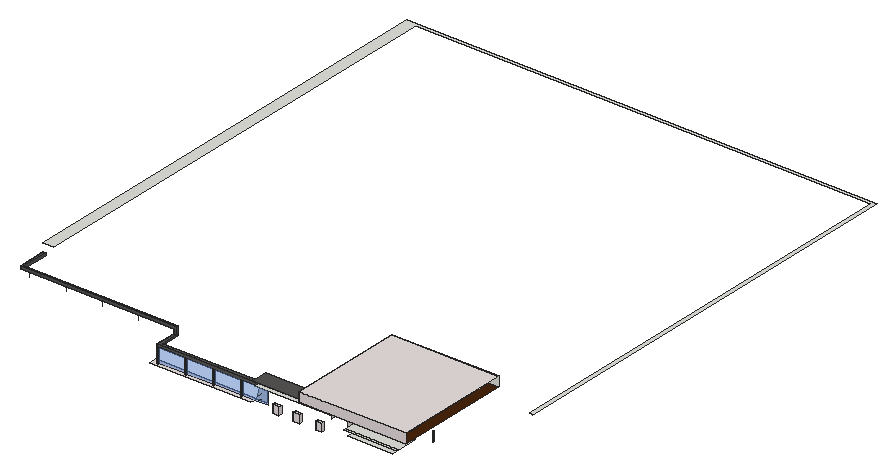
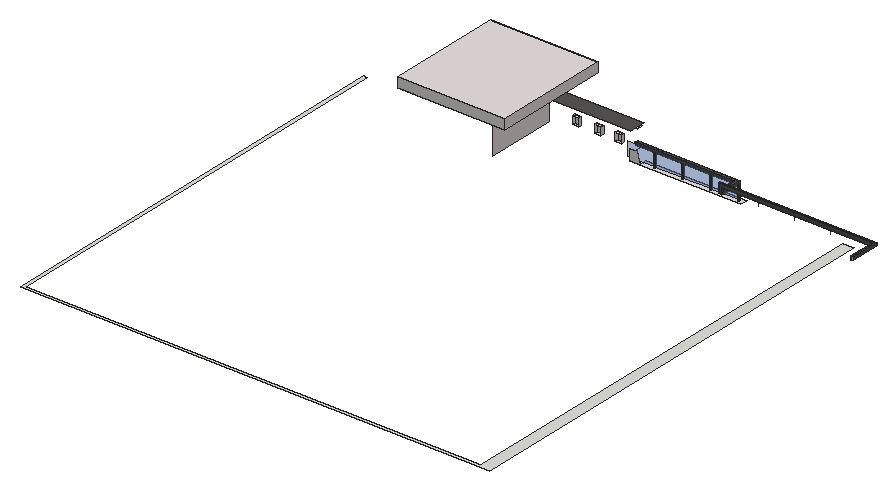
# SketchUp Ruby script. Lengths in inches.
U = 1.inch
M = Sketchup.active_model
def pt(a) = Geom::Point3d.new(a.map { |v| v * U })
def face(e, loops, mat)
  f = e.add_face(loops[0].map { |a| pt(a) })
  loops[1..].each { |l| e.add_face(l.map { |a| pt(a) }).erase! }
  f.material = f.back_material = mat if mat
  f
end
# faces: each face lists its corners as indices into pts; further lists are holes
def faces(e, pts, list, mat = nil) = list.each { |f| face(e, (f[0].is_a?(Array) ? f : [f]).map { |l| l.map { |i| pts[i] } }, mat) }
# xy, xz, yz: faces in a plane at the given z, y or x. An outline is a flat list of corners, or four numbers for a rectangle; further outlines are holes
def ring(l) = l.size == 4 ? [[l[0], l[1]], [l[2], l[1]], [l[2], l[3]], [l[0], l[3]]] : l.each_slice(2).to_a
def flat(e, list, mat, &to3) = list.each { |f| face(e, (f[0].is_a?(Array) ? f : [f]).map { |l| ring(l).map { |u, v| to3.(u, v) } }, mat) }
def xy(e, z, list, mat = nil) = flat(e, list, mat) { |x, y| [x, y, z] }
def xz(e, y, list, mat = nil) = flat(e, list, mat) { |x, z| [x, y, z] }
def yz(e, x, list, mat = nil) = flat(e, list, mat) { |y, z| [x, y, z] }
def lines(e, pts, list) = list.each { |a, b| e.add_line(pt(pts[a]), pt(pts[b])) }
# prism: a flat outline (further loops are holes) pulled along v
def prism(e, loops, v, mat = nil)
  f = face(e, loops, mat); d = Geom::Vector3d.new(v.map { |x| x * U })
  f.pushpull(f.normal.samedirection?(d) ? d.length : -d.length)
end
def box(e, o, s, mat = nil) = prism(e, [[o, [o[0] + s[0], o[1], o[2]], [o[0] + s[0], o[1] + s[1], o[2]], [o[0], o[1] + s[1], o[2]]]], [0, 0, s[2]], mat)
def at(x, y, z, deg = 0) = Geom::Transformation.translation(pt([x, y, z])) * Geom::Transformation.rotation(ORIGIN, Z_AXIS, deg.degrees)
def axes(o, x, y, z) = Geom::Transformation.new([*x, 0, *y, 0, *z, 0, *pt(o).to_a, 1])
def part(name) = M.definitions.add(name)
# library, detail: a bought-in or finely detailed component or shape, given as its bounding box
def library(name, o, s) = part(name).tap { |d| box(d.entities, o, s) }
def detail(e, o, s) = box(e.add_group.entities, o, s)
def put(e, d, t, mat = nil) = e.add_instance(d, t).tap { |i| i.material = mat if mat }
def group(e, t, mat = nil) = e.add_group.tap { |g| g.transformation = t; g.material = mat if mat }.entities
root = M.entities
M.materials.add("Generic\#1").color = [72, 38, 12]
M.materials.add("Generic\#2").color = [87, 84, 84]
M.materials.add("Generic\#9").color = [233, 223, 223]
M.materials.add("[Color M07]").color = [58, 58, 58]
M.materials.add("[Translucent Glass Blue]").color = [100, 149, 237]
M.materials["[Translucent Glass Blue]"].alpha = 0.5
xy(root,250.531,[[[209.664,120.9375,306.609,120.9375,306.609,124.118,296.245,123.803,296.244,123.791,296.175,123.625,296.066,123.482,295.924,123.373,295.758,123.305,295.58,123.281,295.402,123.305,295.236,123.373,295.094,123.482,294.984,123.625,294.916,123.791,294.892,123.969,294.916,124.147,294.984,124.3125,295.094,124.455,295.236,124.564,295.402,124.633,295.58,124.656,295.758,124.633,295.924,124.564,296.066,124.455,296.175,124.3125,296.244,124.147,296.267,123.969,296.245,123.803,306.609,124.118,306.609,127.4375,209.664,127.4375],[268.58,123.281,268.402,123.305,268.236,123.373,268.094,123.482,267.984,123.625,267.916,123.791,267.892,123.969,267.916,124.147,267.941,124.208,267.984,124.3125,268.094,124.455,268.236,124.564,268.402,124.633,268.58,124.656,268.758,124.633,268.924,124.564,269.066,124.455,269.175,124.3125,269.244,124.147,269.267,123.969,269.244,123.791,269.175,123.625,269.066,123.482,268.924,123.373,268.758,123.305],[241.767,123.281,241.589,123.305,241.424,123.373,241.281,123.482,241.172,123.625,241.103,123.791,241.08,123.969,241.103,124.147,241.172,124.3125,241.281,124.455,241.424,124.564,241.589,124.633,241.767,124.656,241.945,124.633,242.111,124.564,242.253,124.455,242.363,124.3125,242.431,124.147,242.455,123.969,242.431,123.791,242.363,123.625,242.253,123.482,242.111,123.373,241.945,123.305],[214.767,123.281,214.589,123.305,214.424,123.373,214.281,123.482,214.172,123.625,214.103,123.791,214.08,123.969,214.103,124.147,214.172,124.3125,214.281,124.455,214.424,124.564,214.589,124.633,214.767,124.656,214.945,124.633,215.111,124.564,215.253,124.455,215.363,124.3125,215.431,124.147,215.455,123.969,215.431,123.791,215.363,123.625,215.253,123.482,215.111,123.373,214.945,123.305]]],"Generic\#9")
xy(root,254.001,[[333.741,113.25,339.991,115.8125],[353.491,113.25,359.741,115.8125],[374.741,113.25,380.991,115.8125]],"Generic\#9")
xy(root,261.564,[[333.741,113.25,339.991,115.8125],[353.491,113.25,359.741,115.8125],[374.741,113.25,380.991,115.8125]],"Generic\#9")
xy(root,264.559,[[411.648,106.0625,454.828,113.125]])
xy(root,265.119,[[[214.101,123.115,214.101,123.807,214.103,123.791,214.172,123.625,214.281,123.482,214.424,123.373,214.589,123.305,214.767,123.281,214.945,123.305,241.589,123.305,241.767,123.281,241.945,123.305,242.363,123.305,242.363,123.625,242.431,123.791,242.455,123.969,242.431,124.147,242.363,124.3125,242.253,124.455,242.111,124.564,241.945,124.633,241.767,124.656,241.589,124.633,241.424,124.564,241.281,124.455,241.172,124.3125,215.363,124.3125,215.253,124.455,215.111,124.564,214.945,124.633,214.767,124.656,214.589,124.633,214.424,124.564,214.281,124.455,214.172,124.3125,214.103,124.147,214.101,124.13,214.101,145.287,217.038,145.287,217.038,126.052,311.912,126.052,311.912,123.115],[295.58,123.281,295.758,123.305,295.924,123.373,296.066,123.482,296.175,123.625,296.244,123.791,296.267,123.969,296.244,124.147,296.175,124.3125,296.066,124.455,295.924,124.564,295.758,124.633,295.58,124.656,295.402,124.633,295.236,124.564,295.094,124.455,294.984,124.3125,294.916,124.147,294.892,123.969,294.916,123.791,294.984,123.625,295.094,123.482,295.236,123.373,295.402,123.305],[268.58,123.281,268.758,123.305,268.924,123.373,269.066,123.482,269.175,123.625,269.244,123.791,269.267,123.969,269.244,124.147,269.175,124.3125,269.066,124.455,268.924,124.564,268.758,124.633,268.58,124.656,268.402,124.633,268.236,124.564,268.094,124.455,267.984,124.3125,267.916,124.147,267.892,123.969,267.916,123.791,267.984,123.625,268.094,123.482,268.236,123.373,268.402,123.305]],[311.912,123.115,312.403,126.052],[214.767,123.281,214.589,123.305,214.945,123.305],[241.767,123.281,241.589,123.305,241.945,123.305],[214.589,123.305,214.424,123.373,214.281,123.482,214.172,123.625,214.103,123.791,214.101,123.807,214.101,124.13,214.103,124.147,214.172,124.3125,214.281,124.455,214.424,124.564,214.589,124.633,214.767,124.656,214.945,124.633,215.111,124.564,215.253,124.455,215.363,124.3125,214.589,124.3125],
  [214.589,123.305,214.589,124.3125,215.363,124.3125,215.431,124.147,215.455,123.969,215.431,123.791,215.363,123.625,215.253,123.482,215.111,123.373,214.945,123.305],[214.945,123.305,215.111,123.373,215.253,123.482,215.363,123.625,215.431,123.791,215.455,123.969,215.431,124.147,215.363,124.3125,241.172,124.3125,241.103,124.147,241.08,123.969,241.103,123.791,241.172,123.625,241.281,123.482,241.424,123.373,241.589,123.305],[241.589,123.305,241.424,123.373,241.281,123.482,241.172,123.625,241.103,123.791,241.08,123.969,241.103,124.147,241.172,124.3125,242.363,124.3125,242.363,123.625,242.253,123.482,242.111,123.373,241.945,123.305],[241.945,123.305,242.111,123.373,242.253,123.482,242.363,123.625,242.363,123.305],[242.363,123.625,242.363,124.3125,242.431,124.147,242.455,123.969,242.431,123.791],
  [214.101,123.807,214.101,124.13,214.08,123.969],[241.172,124.3125,241.281,124.455,241.424,124.564,241.589,124.633,241.767,124.656,241.945,124.633,242.111,124.564,242.253,124.455,242.363,124.3125],[214.101,124.744,213.752,124.79,213.752,127.4375,214.101,127.4375]])
xy(root,267.247,[[214.294,123.307,214.294,143.159,217.231,143.159,217.231,126.245,312.403,126.245,312.403,123.307]],"Generic\#2")
xy(root,268.366,[[407.84,106.0625,458.635,108.375],[407.84,108.375,458.635,127.4375]])
xy(root,271.3125,[[75.429,143.428,75.607,143.451,75.773,143.52,75.915,143.629,76.025,143.771,76.093,143.937,76.117,144.115,76.093,144.293,76.025,144.459,75.915,144.601,75.773,144.711,75.607,144.779,75.429,144.803,75.251,144.779,75.086,144.711,74.943,144.601,74.834,144.459,74.765,144.293,74.742,144.115,74.765,143.937,74.834,143.771,74.943,143.629,75.086,143.52,75.251,143.451],[110.367,143.428,110.545,143.451,110.711,143.52,110.853,143.629,110.962,143.771,111.031,143.937,111.032,143.945,109.703,143.939,109.703,143.937,109.771,143.771,109.881,143.629,110.023,143.52,110.189,143.451],[145.179,143.428,145.357,143.451,145.523,143.52,145.665,143.629,145.775,143.771,145.843,143.937,145.867,144.115,145.866,144.118,144.492,144.112,144.515,143.937,144.584,143.771,144.693,143.629,144.836,143.52,145.001,143.451],[179.992,143.428,180.17,143.451,180.336,143.52,180.478,143.629,180.587,143.771,180.656,143.937,180.679,144.115,180.656,144.291,179.327,144.285,179.304,144.115,179.328,143.937,179.396,143.771,179.506,143.629,179.648,143.52,179.814,143.451],[214.992,143.428,215.17,143.451,215.336,143.52,215.478,143.629,215.587,143.771,215.656,143.937,215.679,144.115,215.656,144.293,215.587,144.459,215.478,144.601,215.336,144.711,215.17,144.779,214.992,144.803,214.955,144.798,214.814,144.779,214.648,144.711,214.506,144.601,214.396,144.459,214.328,144.293,214.304,144.115,214.328,143.937,214.396,143.771,214.506,143.629,214.648,143.52,214.814,143.451,214.955,143.433],
  [109.703,143.939,111.032,143.945,111.054,144.115,111.031,144.293,110.962,144.459,110.853,144.601,110.711,144.711,110.545,144.779,110.367,144.803,110.189,144.779,110.023,144.711,109.881,144.601,109.771,144.459,109.703,144.293,109.679,144.115],[144.492,144.112,145.866,144.118,145.843,144.293,145.775,144.459,145.665,144.601,145.523,144.711,145.357,144.779,145.179,144.803,145.001,144.779,144.836,144.711,144.693,144.601,144.584,144.459,144.515,144.293,144.492,144.115],[179.327,144.285,180.656,144.291,180.656,144.293,180.587,144.459,180.478,144.601,180.336,144.711,180.17,144.779,179.992,144.803,179.814,144.779,179.648,144.711,179.506,144.601,179.396,144.459,179.328,144.293]])
xy(root,272.627,[[317.954,111.75,393.08,115.8125],[393.08,111.75,394.852,115.8125]])
xy(root,276.252,[[315.959,111.75,394.852,127.4375]],"Generic\#2")
xy(root,281.899,[[67.114,170.6875,77.5625,170.6875,77.5625,605.125,515.25,605.125,515.25,194.75,518.6875,194.75,518.6875,607.4375,67.114,607.4375]])
xy(root,288.793,[[470.289,107.5625,470.852,108.375],[394.852,108.375,470.289,127.4375],[470.289,108.375,470.852,120.9375],[394.852,127.4375,470.289,194.75],[394.852,194.75,470.289,202.1875]])
xy(root,288.793,[[376.914,90.3125,376.914,202.1875,394.852,202.1875,394.852,108.375,470.289,108.375,470.289,107.5625,470.852,107.5625,470.852,120.9375,470.289,120.9375,470.289,202.1875,479.727,202.1875,479.727,90.3125]],"Generic\#1")
xy(root,297.793,[[376.914,90.3125,479.727,202.1875]],"Generic\#9")
xz(root,90.3125,[[376.914,288.793,479.727,297.793]],"Generic\#9")
xz(root,113.25,[[333.741,254.001,339.991,261.564],[353.491,254.001,359.741,261.564],[374.741,254.001,380.991,261.564]],"Generic\#9")
xz(root,127.4375,[[306.609,250.531,310.437,261.0625,316.414,261.0625,316.414,250.531]])
xz(root,143.159,[[214.294,267.247,214.294,271.308,67.114,271.308,67.114,274.245,217.231,274.245,217.231,267.247]],"Generic\#2")
xz(root,145.287,[[214.101,265.119,217.038,265.119,217.038,274.052,69.242,274.052,69.242,271.115,214.101,271.115]],"Generic\#2")
xz(root,170.75,[[69.242,271.115,69.242,274.052,67.114,274.245,67.114,271.308]])
xz(root,202.1875,[[376.914,288.793,479.727,297.793]])
yz(root,67.114,[[170.6875,271.308,170.75,274.245]])
yz(root,67.114,[[143.159,271.308,170.6875,274.245]],"Generic\#2")
yz(root,69.242,[[145.287,271.115,170.75,274.052]],"Generic\#2")
yz(root,312.403,[[123.115,265.119,123.237,266.469,123.307,267.247,126.245,267.247,126.175,266.469,126.052,265.119]])
yz(root,333.741,[[113.25,254.001,115.8125,261.564]],"Generic\#9")
yz(root,339.991,[[113.25,254.001,115.8125,261.564]],"Generic\#9")
yz(root,353.491,[[113.25,254.001,115.8125,261.564]],"Generic\#9")
yz(root,359.741,[[113.25,254.001,115.8125,261.564]],"Generic\#9")
yz(root,374.741,[[113.25,254.001,115.8125,261.564]],"Generic\#9")
yz(root,376.914,[[90.3125,288.793,202.1875,297.793]],"Generic\#9")
yz(root,380.991,[[113.25,254.001,115.8125,261.564]],"Generic\#9")
yz(root,394.852,[[108.375,272.627,111.75,276.252],[111.75,272.627,127.4375,276.252]])
yz(root,394.852,[[127.4375,256.5625,127.4375,276.252,108.375,276.252,108.375,288.793,194.75,288.793,194.75,256.5625]],"Generic\#9")
p = [[214.424,123.373,250.531],[214.589,123.305,250.531],[214.589,123.305,265.119],[214.424,123.373,265.119],[214.767,123.281,250.531],[214.767,123.281,265.119],
  [214.945,123.305,250.531],[214.945,123.305,265.119],[215.111,123.373,250.531],[215.111,123.373,265.119],[241.424,123.373,250.531],[241.589,123.305,250.531],
  [241.589,123.305,265.119],[241.424,123.373,265.119],[241.767,123.281,250.531],[241.767,123.281,265.119],[241.945,123.305,250.531],[241.945,123.305,265.119],
  [242.111,123.373,250.531],[242.111,123.373,265.119],[268.236,123.373,250.531],[268.402,123.305,250.531],[268.402,123.305,265.119],[268.236,123.373,265.119],
  [268.58,123.281,250.531],[268.58,123.281,265.119],[268.758,123.305,250.531],[268.758,123.305,265.119],[268.924,123.373,250.531],[268.924,123.373,265.119],
  [295.236,123.373,250.531],[295.402,123.305,250.531],[295.402,123.305,265.119],[295.236,123.373,265.119],[295.58,123.281,250.531],[295.58,123.281,265.119],
  [295.758,123.305,250.531],[295.758,123.305,265.119],[295.924,123.373,250.531],[295.924,123.373,265.119],[214.281,123.482,250.531],[214.281,123.482,265.119],
  [215.253,123.482,250.531],[215.253,123.482,265.119],[215.253,123.432,264.809],[215.253,123.432,250.531],[240.965,124.212,250.531],[240.965,124.212,264.809],
  [241.281,123.482,250.531],[241.281,123.482,265.119],[242.253,123.482,250.531],[242.253,123.482,265.119],[242.378,123.432,264.809],[242.378,123.432,250.531],
  [267.941,124.208,250.531],[268.09,124.212,250.531],[268.09,124.212,264.809],[268.094,123.482,250.531],[268.094,123.482,265.119],[269.066,123.482,250.531],
  [269.066,123.482,265.119],[295.094,123.482,250.531],[295.094,123.482,265.119],[296.066,123.482,250.531],[296.066,123.482,265.119],[214.172,123.625,250.531],
  [214.172,123.625,265.119],[215.363,123.625,250.531],[215.363,123.625,265.119],[241.172,123.625,250.531],[241.172,123.625,265.119],[242.363,123.625,250.531],
  [242.363,123.625,265.119],[267.984,123.625,250.531],[267.984,123.625,265.119],[269.175,123.625,250.531],[269.175,123.625,265.119],[294.984,123.625,250.531],
  [294.984,123.625,265.119],[296.175,123.625,250.531],[296.175,123.625,265.119],[214.103,123.791,250.531],[214.103,123.791,265.119],[215.431,123.791,250.531],
  [215.431,123.791,265.119],[241.103,123.791,250.531],[241.103,123.791,265.119],[242.431,123.791,250.531],[242.431,123.791,265.119],[267.916,123.791,250.531],
  [267.916,123.791,265.119],[269.244,123.791,250.531],[269.244,123.791,265.119],[294.916,123.791,250.531],[294.916,123.791,265.119],[296.244,123.791,250.531],
  [296.244,123.791,265.119],[214.08,123.969,250.531],[214.101,123.807,265.119],[214.08,123.969,265.119],[215.455,123.969,250.531],[215.455,123.969,265.119],
  [241.08,123.969,250.531],[241.08,123.969,265.119],[242.455,123.969,250.531],[242.455,123.969,265.119],[267.892,123.969,250.531],[267.892,123.969,265.119],
  [269.267,123.969,250.531],[269.267,123.969,265.119],[269.286,123.776,264.809],[269.286,123.776,250.531],[294.849,124.552,250.531],[294.998,124.556,250.531],
  [294.998,124.556,264.809],[294.892,123.969,250.531],[294.892,123.969,265.119],[295.348,123.776,264.809],[295.348,123.776,250.531],[296.245,123.803,250.531],
  [306.609,124.118,250.531],[320.912,124.552,250.531],[321.061,124.556,250.531],[321.061,124.556,264.809],[296.267,123.969,250.531],[296.267,123.969,265.119],
  [214.103,124.147,250.531],[214.101,124.13,265.119],[214.103,124.147,265.119],[215.431,124.147,250.531],[215.431,124.147,265.119],[241.103,124.147,250.531],
  [241.103,124.147,265.119],[242.431,124.147,250.531],[242.431,124.147,265.119],[267.916,124.147,250.531],[267.916,124.147,265.119],[269.244,124.147,250.531],
  [269.244,124.147,265.119],[294.916,124.147,250.531],[294.916,124.147,265.119],[296.244,124.147,250.531],[296.244,124.147,265.119],[214.172,124.3125,250.531],
  [214.172,124.3125,265.119],[215.363,124.3125,250.531],[215.363,124.3125,265.119],[241.172,124.3125,250.531],[241.172,124.3125,265.119],[242.363,124.3125,250.531],
  [242.363,124.3125,265.119],[267.984,124.3125,265.119],[267.984,124.3125,250.531],[269.175,124.3125,250.531],[269.175,124.3125,265.119],[294.984,124.3125,250.531],
  [294.984,124.3125,265.119],[296.175,124.3125,250.531],[296.175,124.3125,265.119],[214.281,124.455,250.531],[214.281,124.455,265.119],[215.253,124.455,250.531],
  [215.253,124.455,265.119],[241.281,124.455,250.531],[241.281,124.455,265.119],[242.253,124.455,250.531],[242.253,124.455,265.119],[268.094,124.455,250.531],
  [268.094,124.455,265.119],[269.066,124.455,250.531],[269.066,124.455,265.119],[295.094,124.455,250.531],[295.094,124.455,265.119],[296.066,124.455,250.531],
  [296.066,124.455,265.119],[214.424,124.564,250.531],[214.424,124.564,265.119],[215.111,124.564,250.531],[215.111,124.564,265.119],[241.424,124.564,250.531],
  [241.424,124.564,265.119],[242.111,124.564,250.531],[242.111,124.564,265.119],[268.236,124.564,250.531],[268.236,124.564,265.119],[268.924,124.564,250.531],
  [268.924,124.564,265.119],[295.236,124.564,250.531],[295.236,124.564,265.119],[295.924,124.564,250.531],[295.924,124.564,265.119],[214.589,124.633,250.531],
  [214.589,124.633,265.119],[214.767,124.656,250.531],[214.767,124.656,265.119],[214.945,124.633,250.531],[214.945,124.633,265.119],[241.589,124.633,250.531],
  [241.589,124.633,265.119],[241.767,124.656,250.531],[241.767,124.656,265.119],[241.945,124.633,250.531],[241.945,124.633,265.119],[268.402,124.633,250.531],
  [268.402,124.633,265.119],[268.58,124.656,250.531],[268.58,124.656,265.119],[268.758,124.633,250.531],[268.758,124.633,265.119],[295.402,124.633,250.531],
  [295.402,124.633,265.119],[295.58,124.656,250.531],[295.58,124.656,265.119],[295.758,124.633,250.531],[295.758,124.633,265.119],[214.294,123.307,267.247],
  [214.101,123.115,265.119],[214.101,124.744,265.119],[214.101,127.4375,265.119],[214.101,143.103,265.119],[214.101,145.287,265.119],[214.294,143.159,267.247],
  [295.58,123.115,265.119],[311.912,123.115,265.119],[312.403,123.237,266.469],[312.403,123.307,267.247],[295.58,123.307,267.247],[268.705,123.307,267.247],
  [241.83,123.307,267.247],[241.83,123.115,265.119],[268.705,123.115,265.119],[312.403,123.115,265.119],[217.038,126.052,265.119],[217.231,126.245,267.247],
  [217.231,143.159,267.247],[217.038,145.287,265.119],[312.403,126.245,267.247],[312.403,126.175,266.469],[311.912,126.052,265.119],[295.58,126.052,265.119],
  [268.705,126.052,265.119],[241.83,126.052,265.119],[241.83,126.245,267.247],[268.705,126.245,267.247],[295.58,126.245,267.247],[312.403,126.052,265.119],
  [214.101,145.287,271.115],[214.294,143.159,271.308],[217.231,143.159,274.245],[217.038,145.287,274.052],[67.114,143.159,271.308],[69.242,145.287,271.115],
  [69.242,170.75,271.115],[67.114,170.75,271.308],[67.114,170.6875,271.308],[474.303,129.511,271.312],[474.454,129.448,271.312],[474.454,129.448,280.653],
  [474.303,129.511,280.653],[474.615,129.427,271.312],[474.615,129.427,280.653],[474.777,129.448,271.312],[474.777,129.448,280.653],[474.928,129.511,271.312],
  [474.928,129.511,280.653],[474.173,129.61,271.312],[474.173,129.61,280.653],[475.057,129.61,271.312],[475.057,129.61,280.653],[474.074,129.74,271.312],
  [474.074,129.74,280.653],[475.157,129.74,271.312],[475.157,129.74,280.653],[474.012,129.89,271.312],[474.012,129.89,280.653],[474.012,129.89,279.832],
  [473.99,130.052,271.312],[473.99,130.052,280.653],[474.012,130.214,271.312],[474.012,130.214,280.653],[474.074,130.365,271.312],[474.074,130.365,280.653],
  [475.219,130.214,271.312],[475.157,130.365,271.312],[475.157,130.365,280.653],[475.219,130.214,280.653],[474.173,130.494,271.312],[474.173,130.494,280.653],
  [475.057,130.494,271.312],[475.057,130.494,280.653],[474.303,130.593,271.312],[474.303,130.593,280.653],[474.928,130.593,271.312],[474.928,130.593,280.653],
  [474.454,130.656,271.312],[474.454,130.656,280.653],[474.777,130.656,271.312],[474.777,130.656,280.653],[474.615,130.677,271.312],[474.615,130.677,280.653],
  [69.242,145.287,274.052],[67.114,143.159,274.245],[67.114,170.6875,274.245],[67.114,170.75,274.245],[69.242,170.75,274.052],[316.414,120.9375,261.0625],
  [316.414,115.8125,261.0625],[316.414,120.9375,256.5625],[316.414,115.8125,256.5625],[315.959,115.8125,276.252],[317.954,115.8125,272.627],[394.852,107.5625,288.793],
  [394.852,108.375,288.793],[316.414,127.75,250.531],[316.414,127.4375,250.531],[214.955,123.969,250.531],[214.955,123.969,266.469],[241.83,123.969,266.469],
  [241.83,123.969,250.531],[268.705,123.969,266.469],[268.705,123.969,250.531],[295.58,123.969,266.469],[295.58,123.969,250.531],[312.403,123.969,266.469],
  [214.955,143.433,266.469],[214.955,143.9375,266.469],[214.955,143.9375,271.969],[145.165,143.9375,271.969],[67.892,143.9375,271.969],[67.892,165.5,271.969],
  [180.06,143.9375,266.469],[180.06,143.9375,271.237],[145.165,143.9375,266.469],[145.165,143.9375,272.094],[110.27,143.9375,266.469],[110.27,143.9375,271.237],
  [75.375,143.9375,266.469],[75.375,143.9375,271.237]]
faces(root,p,[[0,1,2,3],[1,4,5,2],[4,6,7,5],[6,8,9,7],[10,11,12,13],[11,14,15,12],[14,16,17,15],[16,18,19,17],
  [20,21,22,23],[21,24,25,22],[24,26,27,25],[26,28,29,27],[30,31,32,33],[31,34,35,32],[34,36,37,35],[36,38,39,37],
  [40,0,3,41],[8,42,43,9],[48,10,13,49],[18,50,51,19],[57,20,23,58],[28,59,60,29],[61,30,33,62],[38,63,64,39],
  [65,40,41,66],[42,67,68,43],[69,48,49,70],[50,71,72,51],[73,57,58,74],[59,75,76,60],[77,61,62,78],[63,79,80,64],
  [81,65,66,82],[67,83,84,68],[85,69,70,86],[71,87,88,72],[89,73,74,90],[75,91,92,76],[93,77,78,94],[79,95,96,80],
  [97,81,82,98,99],[83,100,101,84],[102,85,86,103],[87,104,105,88],[106,89,90,107],[91,108,109,92],[115,93,94,116],[119,124,125,96,95],
  [126,97,99,127,128],[100,129,130,101],[131,102,103,132],[104,133,134,105],[135,106,107,136],[108,137,138,109],[139,115,116,140],[124,141,142,125],
  [143,126,128,144],[129,145,146,130],[147,131,132,148],[133,149,150,134],[54,135,136,151,152],[137,153,154,138],[155,139,140,156],[141,157,158,142],
  [159,143,144,160],[145,161,162,146],[163,147,148,164],[149,165,166,150],[167,152,151,168],[153,169,170,154],[171,155,156,172],[157,173,174,158],
  [175,159,160,176],[161,177,178,162],[179,163,164,180],[165,181,182,166],[183,167,168,184],[169,185,186,170],[187,171,172,188],[173,189,190,174],
  [191,175,176,192],[193,191,192,194],[195,193,194,196],[177,195,196,178],[197,179,180,198],[199,197,198,200],[201,199,200,202],[181,201,202,182],
  [203,183,184,204],[205,203,204,206],[207,205,206,208],[185,207,208,186],[209,187,188,210],[211,209,210,212],[213,211,212,214],[189,213,214,190],
  [215,216,98,127,217,218,219,220,221],[222,223,224,225,226,227,228,215,216,229,230],[232,233,234,235],[236,237,238,239,240,241,232,233,242,243,244],[221,220,246,247],[235,234,248,249],[300,301,302,303,304],[249,248,301,300]],"Generic\#2")
faces(root,p,[[44,45,46,47],[52,53,54,55,56],[110,111,112,113,114],[117,118,119,120,121,122,123]],"[Translucent Glass Blue]")
faces(root,p,[[224,231,223],[238,245,237],[250,251,252,253,254],[247,246,251,250]])
faces(root,p,[[255,256,257,258],[256,259,260,257],[259,261,262,260],[261,263,264,262],[265,255,258,266],[263,267,268,264],[269,265,266,270],[267,271,272,268],
  [273,269,270,274,275],[276,273,275,274,277],[278,276,277,279],[280,278,279,281],[282,283,284,285],[286,280,281,287],[283,288,289,284],[290,286,287,291],
  [288,292,293,289],[294,290,291,295],[292,296,297,293],[298,294,295,299],[296,298,299,297]],"[Color M07]")
lines(root,p,[[305,306],[307,308],[309,310],[311,312],[313,314],[315,316],[316,317],[318,317],[317,319],[320,319],[319,321],[322,321],
  [321,323],[316,324],[325,326],[326,327],[328,329],[330,331],[332,327],[327,328],[327,333],[334,335],[336,337],[324,325]])
